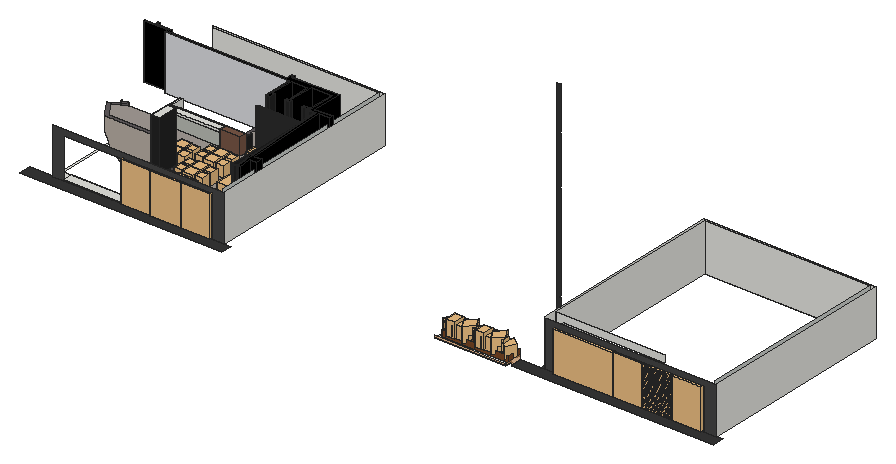
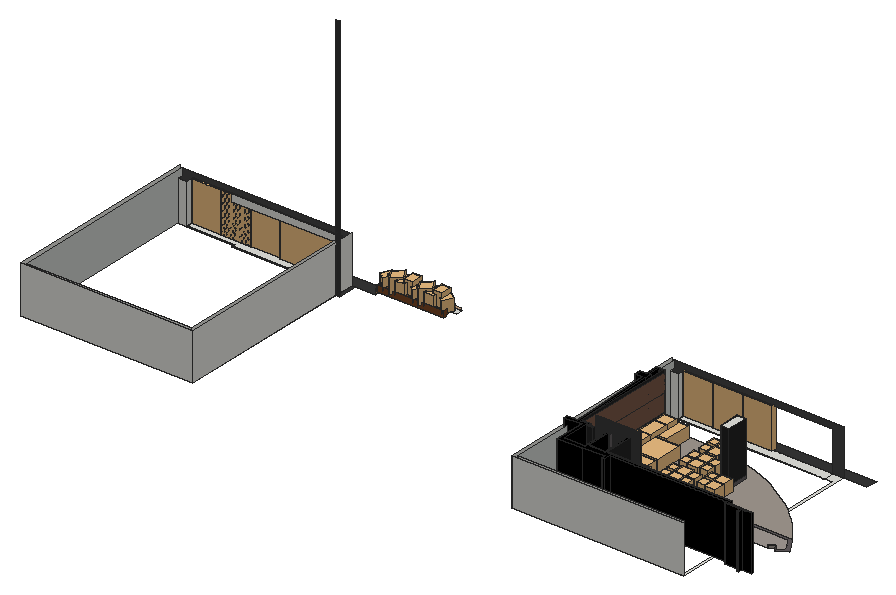
# SketchUp Ruby script. Lengths in inches.
U = 1.inch
M = Sketchup.active_model
def pt(a) = Geom::Point3d.new(a.map { |v| v * U })
def face(e, loops, mat)
  f = e.add_face(loops[0].map { |a| pt(a) })
  loops[1..].each { |l| e.add_face(l.map { |a| pt(a) }).erase! }
  f.material = f.back_material = mat if mat
  f
end
# faces: each face lists its corners as indices into pts; further lists are holes
def faces(e, pts, list, mat = nil) = list.each { |f| face(e, (f[0].is_a?(Array) ? f : [f]).map { |l| l.map { |i| pts[i] } }, mat) }
# xy, xz, yz: faces in a plane at the given z, y or x. An outline is a flat list of corners, or four numbers for a rectangle; further outlines are holes
def ring(l) = l.size == 4 ? [[l[0], l[1]], [l[2], l[1]], [l[2], l[3]], [l[0], l[3]]] : l.each_slice(2).to_a
def flat(e, list, mat, &to3) = list.each { |f| face(e, (f[0].is_a?(Array) ? f : [f]).map { |l| ring(l).map { |u, v| to3.(u, v) } }, mat) }
def xy(e, z, list, mat = nil) = flat(e, list, mat) { |x, y| [x, y, z] }
def xz(e, y, list, mat = nil) = flat(e, list, mat) { |x, z| [x, y, z] }
def yz(e, x, list, mat = nil) = flat(e, list, mat) { |y, z| [x, y, z] }
def lines(e, pts, list) = list.each { |a, b| e.add_line(pt(pts[a]), pt(pts[b])) }
# prism: a flat outline (further loops are holes) pulled along v
def prism(e, loops, v, mat = nil)
  f = face(e, loops, mat); d = Geom::Vector3d.new(v.map { |x| x * U })
  f.pushpull(f.normal.samedirection?(d) ? d.length : -d.length)
end
def box(e, o, s, mat = nil) = prism(e, [[o, [o[0] + s[0], o[1], o[2]], [o[0] + s[0], o[1] + s[1], o[2]], [o[0], o[1] + s[1], o[2]]]], [0, 0, s[2]], mat)
def at(x, y, z, deg = 0) = Geom::Transformation.translation(pt([x, y, z])) * Geom::Transformation.rotation(ORIGIN, Z_AXIS, deg.degrees)
def axes(o, x, y, z) = Geom::Transformation.new([*x, 0, *y, 0, *z, 0, *pt(o).to_a, 1])
def part(name) = M.definitions.add(name)
# library, detail: a bought-in or finely detailed component or shape, given as its bounding box
def library(name, o, s) = part(name).tap { |d| box(d.entities, o, s) }
def detail(e, o, s) = box(e.add_group.entities, o, s)
def put(e, d, t, mat = nil) = e.add_instance(d, t).tap { |i| i.material = mat if mat }
def group(e, t, mat = nil) = e.add_group.tap { |g| g.transformation = t; g.material = mat if mat }.entities
root = M.entities
M.materials.add("Biselado").color = [218, 219, 223]
M.materials.add("Concrete").color = [186, 188, 181]
M.materials.add("Floor board").color = [119, 86, 70]
M.materials.add("Floor board2").color = [119, 86, 70]
M.materials.add("Material__1").color = [95, 70, 46]
M.materials.add("Plastic Black ").color = [43, 43, 43]
M.materials.add("Screen Shot 2014-10-30 at 12.13.07").color = [162, 155, 149]
M.materials.add("Sophie_Shoes2").color = [35, 35, 35]
M.materials.add("Sophie_Skirt").color = [0, 0, 0]
M.materials.add("Untitsled-1").color = [96, 91, 93]
M.materials.add("Wood_Grain_Dark").color = [51, 47, 43]
M.materials.add("[Basic Tile]").color = [203, 206, 202]
M.materials.add("[Color_000]").color = [255, 255, 255]
M.materials.add("[Granite Dark Gray]").color = [69, 68, 68]
M.materials.add("[Metal_Corrogated_Shiny]2").color = [193, 193, 193]
M.materials.add("[Slate Light Tile]").color = [54, 54, 54]
M.materials.add("[Wood Floor]").color = [224, 152, 88]
M.materials["[Wood Floor]"].alpha = 0.68
M.materials.add("[Wood Veneer 01]").color = [120, 70, 37]
M.materials.add("t_planksnew0027_5_l_seamless_298 copy").color = [161, 153, 144]
c1 = library("Square table",[5.01,5.91,-0.2],[27.56,27.56,29.53])
c2 = library("ch24 wishbone chair by Carl Hansen & Son",[0,0,0],[21.1,19.68,29.02])
c3 = library("Scandinavian Door w/ Glass Wall\#2",[-41.94,78.85,0],[6.47,62.99,82.68])
c4 = part("Group\#72")
box(c4.entities,[0,-0.59,0],[31.5,1.77,87.4],"Sophie_Shoes2")
c5 = library("Armless sofa",[0,0,0],[31.59,51.18,39.76])
c6 = library("Sofa corner unit",[0,0,0],[31.57,31.52,39.76])
c7 = part("Group\#13")
box(c7.entities,[-0.79,0,0],[1.97,3.15,131.5],"Wood_Grain_Dark")
c8 = library("Group\#91",[-37.8,-0.03,0],[93.74,69.5,29.53])
c9 = library("Group\#68",[-37.8,-0.03,0],[93.74,69.5,29.53])
c10 = library("Group\#95",[0,-0.03,0],[55.94,69.5,29.53])
c11 = library("Areca palm plant",[0,0,0],[49.1,36.6,54.46])
c12 = library("Group\#440",[-84.69,-90.07,-0.36],[176.51,175.13,171.4])
c13 = library("Group\#441",[-7.34,-1.2,0],[38.67,35.81,49.04])
c14 = library("Group38\#2",[14.01,28.44,-23.43],[18.58,18.32,38.89])
c15 = library("Group20\#1",[-20.81,-17.08,3.79],[39.86,39.43,37.51])
c16 = part("Group\#443")
put(c16.entities,c11,axes([76.39,-6.2,6.08],[0.56191,0.45017,0],[-0.52986,0.66137,0],[0,0,0.72]))
put(c16.entities,c11,axes([178.2,-6.2,6.08],[0.56191,0.45017,0],[-0.52986,0.66137,0],[0,0,0.72]))
put(c16.entities,c12,axes([163.5,14.93,6.05],[0.08593,-0.04961,0],[0.04961,0.08593,0],[0,0,0.10522]))
put(c16.entities,c13,axes([144.89,24.9375,8],[-0.79,0,0],[0,-0.79,0],[0,0,0.79]))
put(c16.entities,c12,axes([113.57,17.19,6.07],[0.14087,-0.08133,0],[0.08133,0.14087,0],[0,0,0.1725]))
put(c16.entities,c14,axes([235.95,-4.1,28.17],[0,0.8848,0],[-0.94674,0,0],[0,0,0.85826]))
put(c16.entities,c12,axes([190.75,14.93,6.05],[0.08593,-0.04961,0],[0.04961,0.08593,0],[0,0,0.10522]))
put(c16.entities,c12,axes([61.68,14.93,6.05],[0.08593,-0.04961,0],[0.04961,0.08593,0],[0,0,0.10522]))
put(c16.entities,c12,axes([88.93,14.93,6.05],[0.08593,-0.04961,0],[0.04961,0.08593,0],[0,0,0.10522]))
put(c16.entities,c15,axes([154.82,18.97,4.77],[-0.85,0,0],[0,-0.85,0],[0,0,0.85]))
put(c16.entities,c12,axes([41.62,14.93,6.05],[0.08593,-0.04961,0],[0.04961,0.08593,0],[0,0,0.10522]))
put(c16.entities,c12,axes([143.43,14.93,6.05],[0.08593,-0.04961,0],[0.04961,0.08593,0],[0,0,0.10522]))
put(c16.entities,c14,axes([134.14,-4.1,28.17],[0,0.8848,0],[-0.94674,0,0],[0,0,0.85826]))
g1 = group(c16.entities,at(234.8,0,0,90),"[Wood Veneer 01]")
xy(g1,0,[[0,0,6,234.8],[30,0,36,234.8]])
xy(g1,3,[[6,0,30,234.8]])
xy(g1,7,[[6,5,30,229.8]],"Material__1")
xy(g1,15,[[[0,0,36,234.8],[6,5,30,229.8]]])
xz(g1,0,[[0,0,6,0,6,3,30,3,30,0,36,0,36,15,0,15]])
xz(g1,5,[[6,7,30,15]])
xz(g1,229.8,[[6,7,30,15]])
xz(g1,234.8,[[0,0,0,15,36,15,36,0,30,0,30,3,6,3,6,0]])
yz(g1,0,[[0,0,234.8,15]])
yz(g1,6,[[0,0,234.8,3],[5,7,229.8,15]])
yz(g1,30,[[0,0,234.8,3],[5,7,229.8,15]])
yz(g1,36,[[0,0,234.8,15]])
put(c16.entities,c13,axes([43.08,24.9375,8],[-0.79,0,0],[0,-0.79,0],[0,0,0.79]))
put(c16.entities,c12,axes([11.76,17.19,6.07],[0.14087,-0.08133,0],[0.08133,0.14087,0],[0,0,0.1725]))
put(c16.entities,c15,axes([53.01,18.97,4.77],[-0.85,0,0],[0,-0.85,0],[0,0,0.85]))
put(c16.entities,c12,axes([219.01,17.19,6.07],[0.14087,-0.08133,0],[0.08133,0.14087,0],[0,0,0.1725]))
xy(root,148.4375,[[3053.01,589.17,3053.01,1096.5,3491.44,1096.5,3491.44,589.17,3457.61,589.17,3457.61,608.75,3480.67,608.75,3480.67,1090.24,3059.27,1090.24,3059.27,616,3079.62,616,3079.62,589.17],[3079.62,589.17,3079.62,616,3336.64,616,3336.64,608.75,3457.61,608.75,3457.61,589.17],[4303.63,589.17,4303.63,1096.5,4742.06,1096.5,4742.06,589.17,4708.23,589.17,4708.23,608.75,4731.3,608.75,4731.3,1090.24,4309.9,1090.24,4309.9,616,4330.25,616,4330.25,589.17],[4330.25,589.17,4330.25,616,4587.26,616,4587.26,608.75,4708.23,608.75,4708.23,589.17]])
xy(root,148.4375,[[2993.46,559.875,3506.75,589.17],[4244.09,559.875,4757.37,589.17],[4294.9,589.17,4303.63,640.11]],"[Slate Light Tile]")
xy(root,149.625,[[3079.62,589.17,3457.61,589.17,3457.61,608.75,3336.64,608.75,3336.64,616,3079.62,616],[4330.25,589.17,4708.23,589.17,4708.23,608.75,4587.26,608.75,4587.26,616,4330.25,616]])
xy(root,155.3125,[[4061.87,542.125,4244.09,559.875]])
xz(root,542.125,[[4061.87,155.3125,4244.09,161.375]],"[Wood Floor]")
xz(root,589.17,[[3079.62,148.4375,3336.64,149.625],[3336.64,148.4375,3457.61,149.625],[4330.25,148.4375,4587.26,149.625],[4587.26,148.4375,4708.23,149.625]])
xz(root,589.17,[[3053.01,148.4375,3079.62,148.4375,3079.62,251.46,3457.61,251.46,3457.61,148.4375,3491.44,148.4375,3491.44,265.8125,3053.01,265.8125],[4303.63,148.4375,4330.25,148.4375,4330.25,251.46,4708.23,251.46,4708.23,148.4375,4742.06,148.4375,4742.06,265.8125,4303.63,265.8125]],"[Granite Dark Gray]")
xz(root,608.75,[[3336.64,148.4375,3457.61,149.625],[3457.61,148.4375,3480.67,251.46],[4587.26,148.4375,4708.23,149.625],[4708.23,148.4375,4731.3,251.46]])
xz(root,616,[[3079.62,148.4375,3336.64,149.625],[4309.9,148.4375,4309.9,268.4375,4587.26,268.4375,4587.26,251.46,4330.25,251.46,4330.25,148.4375],[4330.25,148.4375,4587.26,149.625]])
xz(root,640.11,[[4294.9,148.4375,4303.63,148.4375,4303.63,289.5625,4300.2,289.5625,4300.2,293,4303.63,293,4303.63,410.625,4301.7,410.625,4301.7,413.5,4303.63,413.5,4303.63,538.1875,4301.88,538.1875,4301.88,541.1875,4303.63,541.1875,4303.63,662.4375,4301.76,662.4375,4301.76,665.9375,4303.63,665.9375,4303.63,776.0625,4294.9,776.0625]],"[Slate Light Tile]")
xz(root,1090.24,[[3059.27,148.4375,3480.67,268.4375],[4309.9,148.4375,4731.3,268.4375]])
xz(root,1096.5,[[3053.01,148.4375,3491.44,268.4375],[4303.63,148.4375,4742.06,268.4375]])
yz(root,3336.64,[[608.75,148.4375,616,149.625]])
yz(root,3457.61,[[589.17,148.4375,608.75,149.625],[589.17,149.625,608.75,251.46]])
yz(root,3480.67,[[608.75,148.4375,608.75,251.46,595.44,251.46,595.44,268.4375,1090.24,268.4375,1090.24,148.4375]],"[Basic Tile]")
yz(root,3491.44,[[589.17,148.4375,1096.5,268.4375]])
yz(root,4244.09,[[559.875,148.4375,589.17,148.4375,589.17,161.375,542.125,161.375,542.125,155.3125,559.875,155.3125]],"[Wood Floor]")
yz(root,4303.63,[[589.17,148.4375,640.11,268.4375],[640.11,148.4375,1096.5,268.4375]])
yz(root,4309.9,[[616,148.4375,1090.24,268.4375]])
yz(root,4330.25,[[589.17,148.4375,616,149.625],[589.17,149.625,616,251.46]])
yz(root,4587.26,[[608.75,148.4375,616,149.625]])
yz(root,4708.23,[[589.17,148.4375,608.75,149.625],[589.17,149.625,608.75,251.46]])
yz(root,4731.3,[[608.75,148.4375,608.75,251.46,595.44,251.46,595.44,268.4375,1090.24,268.4375,1090.24,148.4375]],"[Basic Tile]")
yz(root,4742.06,[[589.17,148.4375,1096.5,268.4375]])
p = [[3382.97,998.54,148.89],[3382.97,998.73,148.89],[3464.42,662.13,148.89],[3464.46,662.13,148.89],[3451.42,661.28,148.89],[3451.42,661.28,235.5]]
lines(root,p,[[0,1],[2,3],[4,5]])
g2 = group(root,at(3111.07,900.11,148.89))
g3 = group(g2,at(0,0,0))
box(g3,[-5.91,0,0],[163.69,19.69,31.5])
g4 = group(root,at(2948.875,845,148.89),"Untitsled-1")
xy(g4,0,[[30.66,0,22.97,10.41,13.17,25.17,0,47.23,25.07,61.99,28.66,54.97,10.82,44.46,19.84,29.37,29.42,14.93,34.63,7.875,502.55,7.875,502.55,0],[29.6875,52.96,28.66,54.97,25.07,61.99,25.45,62.21,29.03,55.19,29.87,53.55,30.06,53.17],[150.39,55.12,162.2,61.02]])
xy(g4,0,[[34.63,7.875,29.42,14.93,19.84,29.37,10.82,44.46,28.66,54.97,29.6875,52.96,30.06,53.17,43.36,60.59,43.25,60.59,43.25,61.02,150.39,61.02,150.39,55.12,295.57,55.12,295.57,74.8,303.44,74.8,303.44,147.64,382.18,147.64,382.18,74.8,392.39,74.8,392.39,88.58,388.09,88.58,388.09,147.64,428.18,147.64,428.18,88.58,423.88,88.58,423.88,82.68,436.24,82.68,436.24,88.58,434.09,88.58,434.09,153.54,485.64,153.54,485.64,88.58,467.74,88.58,467.74,82.68,480.91,82.68,480.91,79.03,503.34,79.03,503.34,31.5,502.55,31.5,502.55,7.875]],"Screen Shot 2014-10-30 at 12.13.07")
xy(g4,0,[[295.57,74.8,303.44,147.64]],"Untitsled-1")
xy(g4,7.875,[[29.6875,52.96,25.07,61.99,25.45,62.21,29.03,55.19,29.87,53.55,43.25,61.02,43.25,60.59,43.36,60.59]],"Untitsled-1")
xz(g4,60.59,[[43.25,0,43.36,7.875]],"Screen Shot 2014-10-30 at 12.13.07")
yz(g4,43.25,[[60.59,0,61.02,7.875]],"Screen Shot 2014-10-30 at 12.13.07")
p = [[29.6875,52.96,7.875],[25.07,61.99,7.875],[25.07,61.99,0],[28.66,54.97,0],[29.6875,52.96,0],[30.06,53.17,0],
  [43.36,60.59,0],[43.36,60.59,7.875],[29.87,53.55,0],[29.03,55.19,0],[29.03,55.19,7.875],[29.87,53.55,7.875],
  [43.25,61.02,0],[43.25,61.02,7.875],[25.45,62.21,0],[25.45,62.21,7.875],[150.39,55.12,0],[150.39,39.37,0],
  [502.55,0,0],[503.34,0,0],[29.44,55.42,0],[43.45,60.64,0],[25.07,62,0],[502.55,78.21,0],
  [480.91,78.21,0],[480.91,79.03,0],[303.44,147.64,0],[303.44,155.51,0]]
faces(g4,p,[[0,1,2,3,4],[4,5,6,7,0],[8,9,10,11],[9,14,15,10],[14,2,1,15]])
faces(g4,p,[[8,12,13,11]],"Screen Shot 2014-10-30 at 12.13.07")
lines(g4,p,[[16,17],[18,19],[20,9],[6,21],[22,2],[23,24],[24,25],[26,27]])
g5 = group(g4,at(388.09,147.64,0))
xy(g5,0,[[0,-59.06,4.3,-59.06,4.3,-58.62,0.43,-58.62,0.43,-0.43,39.67,-0.43,39.67,-58.62,35.8,-58.62,35.8,-59.06,40.1,-59.06,40.1,0,0,0]],"Screen Shot 2014-10-30 at 12.13.07")
xy(g5,7.875,[[0,-59.06,0,-0.43,0.43,-0.43,0.43,-58.62,4.3,-58.62,4.3,-59.06],[35.8,-59.06,35.8,-58.62,39.67,-58.62,39.67,-0.43,40.1,-0.43,40.1,-59.06]],"Untitsled-1")
xy(g5,47.24,[[0,-0.43,40.1,0]],"Untitsled-1")
xz(g5,-59.06,[[35.8,0,40.1,7.875]],"Screen Shot 2014-10-30 at 12.13.07")
xz(g5,-59.06,[[0,0,4.3,7.875]],"Untitsled-1")
xz(g5,-58.62,[[0.43,0,4.3,7.875],[35.8,0,39.67,7.875]],"Untitsled-1")
xz(g5,-0.43,[[0,7.875,40.1,39.37]],"Screen Shot 2014-10-30 at 12.13.07")
xz(g5,-0.43,[[0.43,0,39.67,7.875],[0,39.37,40.1,47.24]],"Untitsled-1")
yz(g5,0,[[-59.06,0,0,0,0,39.37,-0.43,39.37,-0.43,7.875,-59.06,7.875]],"Screen Shot 2014-10-30 at 12.13.07")
yz(g5,0,[[-0.43,39.37,0,47.24]],"Untitsled-1")
yz(g5,0.43,[[-58.62,0,-0.43,7.875]],"Untitsled-1")
yz(g5,4.3,[[-59.06,0,-58.62,7.875]],"Untitsled-1")
yz(g5,35.8,[[-59.06,0,-58.62,7.875]],"Untitsled-1")
yz(g5,39.67,[[-58.62,0,-0.43,7.875]],"Untitsled-1")
yz(g5,40.1,[[-59.06,0,-59.06,7.875,-0.43,7.875,-0.43,39.37,0,39.37,0,0]],"Screen Shot 2014-10-30 at 12.13.07")
yz(g5,40.1,[[-0.43,39.37,0,47.24]],"Untitsled-1")
g6 = group(g4,at(434.09,153.54,0))
xy(g6,0,[[0,-64.96,2.15,-64.96,2.15,-64.53,0.43,-64.53,0.43,-0.43,51.11,-0.43,51.11,-64.53,33.65,-64.53,33.65,-64.96,51.55,-64.96,51.55,0,0,0]],"Screen Shot 2014-10-30 at 12.13.07")
xy(g6,7.875,[[0,-64.96,0,-0.43,0.43,-0.43,0.43,-64.53,2.15,-64.53,2.15,-64.96],[33.65,-64.96,33.65,-64.53,51.11,-64.53,51.11,-0.43,51.55,-0.43,51.55,-64.96]],"Untitsled-1")
xy(g6,47.24,[[0,-0.43,51.55,0]],"Untitsled-1")
xz(g6,-64.96,[[0,0,2.15,7.875],[33.65,0,51.55,7.875]],"Untitsled-1")
xz(g6,-64.53,[[0.43,0,2.15,7.875],[33.65,0,51.11,7.875]],"Untitsled-1")
xz(g6,-0.43,[[0,7.875,51.55,39.37]],"Screen Shot 2014-10-30 at 12.13.07")
xz(g6,-0.43,[[0.43,0,51.11,7.875],[0,39.37,51.55,47.24]],"Untitsled-1")
xz(g6,0,[[40.1,0,51.55,39.37]],"Screen Shot 2014-10-30 at 12.13.07")
xz(g6,0,[[40.1,39.37,51.55,47.24]],"Untitsled-1")
yz(g6,0,[[-64.96,0,0,0,0,39.37,-0.43,39.37,-0.43,7.875,-64.96,7.875]],"Screen Shot 2014-10-30 at 12.13.07")
yz(g6,0,[[-0.43,39.37,0,47.24]],"Untitsled-1")
yz(g6,0.43,[[-64.53,0,-0.43,7.875]],"Untitsled-1")
yz(g6,2.15,[[-64.96,0,-64.53,7.875]],"Untitsled-1")
yz(g6,33.65,[[-64.96,0,-64.53,7.875]],"Untitsled-1")
yz(g6,51.11,[[-64.53,0,-0.43,7.875]],"Untitsled-1")
yz(g6,51.55,[[-64.96,0,-64.96,7.875,-0.43,7.875,-0.43,39.37,0,39.37,0,0]],"Screen Shot 2014-10-30 at 12.13.07")
yz(g6,51.55,[[-0.43,39.37,0,47.24]],"Untitsled-1")
put(root,c1,at(3223.26,766.11,148.89,89.836))
put(root,c1,at(3223.26,794.18,148.89,89.836))
g7 = group(root,at(3202.39,714.02,148.89))
xy(g7,0,[[-0.59,-0.59,22.24,53.74]])
xy(g7,7.875,[[-0.59,-0.59,22.24,0],[-0.59,0,0,53.15],[21.65,0,22.24,53.15],[-0.59,53.15,22.24,53.74]],"Untitsled-1")
xy(g7,137.44,[[0,0,21.65,53.15]])
xz(g7,-0.59,[[-0.59,0,22.24,7.875]],"Untitsled-1")
xz(g7,0,[[0,7.875,21.65,137.44]],"Sophie_Shoes2")
xz(g7,53.15,[[0,7.875,21.65,137.44]],"Sophie_Shoes2")
xz(g7,53.74,[[-0.59,0,22.24,7.875]],"Untitsled-1")
yz(g7,-0.59,[[-0.59,0,53.74,7.875]],"Untitsled-1")
yz(g7,0,[[0,7.875,53.15,137.44]],"Sophie_Shoes2")
yz(g7,21.65,[[0,7.875,53.15,137.44]],"Sophie_Shoes2")
yz(g7,22.24,[[-0.59,0,53.74,7.875]],"Untitsled-1")
g8 = group(root,at(2952.73,661.35,148.89))
xy(g8,0,[[511.73,0,511.7,0.79,510.27,31.46,508.31,31.46,507.48,49.07,509.45,49.07,499.49,263.4,481.79,262.65,481.79,265.89,463.89,265.89,463.89,272.23,481.79,272.23,481.79,337.19,430.24,337.19,430.24,272.23,432.39,272.23,432.39,265.89,420.03,265.89,420.03,272.23,424.33,272.23,424.33,331.29,384.24,331.29,384.24,272.23,388.54,272.23,388.54,258.02,377.9,258.02,377.9,331.29,62.06,331.29,62.06,341.13,1.14,341.13,0,345.07,25.02,345.07,25.02,355.33,28.95,355.33,28.95,347.03,67.96,347.03,67.96,339.16,365.84,339.16,365.84,355.33,373.72,355.33,373.72,346.57,430.24,349.18,491.63,352.02,491.63,272.99,534.09,274.79,534.09,264.94,507.35,263.81,517.3125,49.53,534.09,50.31,534.09,32.57,518.14,31.83,519.6,0.37,514.8125,0]],"Sophie_Skirt")
xy(g8,7.875,[[377.9,258.02,378.33,331.29],[378.33,258.02,388.54,258.45],[420.03,265.89,432.39,266.33],[463.89,265.89,481.79,266.33]],"Untitsled-1")
xy(g8,137.8,[[511.73,0,514.8125,0,519.6,0.37,518.14,31.83,534.09,32.57,534.09,50.31,517.3125,49.53,507.35,263.81,534.09,264.94,534.09,274.79,491.63,272.99,491.63,352.02,430.24,349.18,373.72,346.57,373.72,355.33,365.84,355.33,365.84,339.16,67.96,339.16,67.96,347.03,28.95,347.03,28.95,355.33,25.02,355.33,25.02,345.07,0,345.07,1.14,341.13,62.06,341.13,62.06,331.29,378.33,331.29,378.33,258.45,388.54,258.45,388.54,272.23,384.24,272.23,384.24,331.29,424.33,331.29,424.33,272.23,420.03,272.23,420.03,266.33,432.39,266.33,432.39,272.23,430.24,272.23,430.24,337.19,481.79,337.19,481.79,272.23,463.89,272.23,463.89,266.33,481.79,266.33,481.79,262.65,499.49,263.4,509.45,49.07,507.48,49.07,508.31,31.46,510.27,31.46,511.7,0.79]],"Sophie_Skirt")
xz(g8,0,[[511.73,0,514.8125,137.8]],"Sophie_Skirt")
xz(g8,31.46,[[508.31,0,510.27,137.8]],"Sophie_Skirt")
xz(g8,49.07,[[507.48,0,509.45,137.8]],"Sophie_Skirt")
xz(g8,258.02,[[377.9,0,388.54,7.875]],"Untitsled-1")
xz(g8,258.45,[[378.33,7.875,388.54,137.8]],"Sophie_Shoes2")
xz(g8,265.89,[[420.03,0,432.39,7.875],[463.89,0,481.79,7.875]],"Untitsled-1")
xz(g8,266.33,[[420.03,7.875,432.39,137.8],[463.89,7.875,481.79,137.8]],"Sophie_Shoes2")
xz(g8,272.23,[[384.24,0,388.54,137.8],[420.03,0,424.33,137.8],[430.24,0,432.39,137.8],[463.89,0,481.79,137.8]],"Sophie_Shoes2")
xz(g8,331.29,[[62.06,0,377.9,0,377.9,7.875,378.33,7.875,378.33,137.8,62.06,137.8]],"Biselado")
xz(g8,331.29,[[384.24,0,424.33,137.8]],"Sophie_Skirt")
xz(g8,337.19,[[430.24,0,481.79,137.8]],"Sophie_Skirt")
xz(g8,339.16,[[67.96,0,365.84,137.8]],"Sophie_Skirt")
xz(g8,341.13,[[1.14,0,62.06,137.8]],"Sophie_Skirt")
xz(g8,345.07,[[0,0,25.02,137.8]],"Sophie_Skirt")
xz(g8,347.03,[[28.95,0,67.96,137.8]],"Sophie_Skirt")
xz(g8,355.33,[[25.02,0,28.95,137.8],[365.84,0,373.72,137.8]],"Sophie_Skirt")
yz(g8,25.02,[[345.07,0,355.33,137.8]],"Sophie_Skirt")
yz(g8,28.95,[[347.03,0,355.33,137.8]],"Sophie_Skirt")
yz(g8,62.06,[[331.29,0,341.13,137.8]],"Sophie_Skirt")
yz(g8,67.96,[[339.16,0,347.03,137.8]],"Sophie_Skirt")
yz(g8,365.84,[[339.16,0,355.33,137.8]],"Sophie_Skirt")
yz(g8,373.72,[[346.57,0,355.33,137.8]],"Sophie_Skirt")
yz(g8,377.9,[[258.02,0,331.29,7.875]],"Untitsled-1")
yz(g8,378.33,[[258.45,7.875,331.29,137.8]],"Sophie_Shoes2")
yz(g8,384.24,[[272.23,0,331.29,137.8]],"Sophie_Skirt")
yz(g8,388.54,[[258.02,0,272.23,0,272.23,137.8,258.45,137.8,258.45,7.875,258.02,7.875]],"Sophie_Shoes2")
yz(g8,420.03,[[265.89,0,265.89,7.875,266.33,7.875,266.33,137.8,272.23,137.8,272.23,0]],"Untitsled-1")
yz(g8,424.33,[[272.23,0,331.29,137.8]],"Sophie_Skirt")
yz(g8,430.24,[[272.23,0,337.19,137.8]],"Sophie_Skirt")
yz(g8,432.39,[[265.89,0,272.23,0,272.23,137.8,266.33,137.8,266.33,7.875,265.89,7.875]],"Sophie_Shoes2")
yz(g8,463.89,[[265.89,0,265.89,7.875,266.33,7.875,266.33,137.8,272.23,137.8,272.23,0]],"Sophie_Shoes2")
yz(g8,481.79,[[262.65,0,262.65,137.8,266.33,137.8,266.33,7.875,265.89,7.875,265.89,0],[272.23,0,337.19,137.8]],"Sophie_Skirt")
yz(g8,491.63,[[272.99,0,352.02,137.8]],"Sophie_Skirt")
yz(g8,534.09,[[32.57,0,50.31,137.8],[264.94,0,274.79,137.8]],"Sophie_Skirt")
p = [[511.7,0.79,0],[511.73,0,0],[511.73,0,137.8],[511.7,0.79,137.8],[514.8125,0,0],[519.6,0.37,0],
  [519.6,0.37,137.8],[514.8125,0,137.8],[518.14,31.83,0],[518.14,31.83,137.8],[510.27,31.46,0],[510.27,31.46,137.8],
  [507.48,49.07,0],[508.31,31.46,0],[508.31,31.46,137.8],[507.48,49.07,137.8],[534.09,32.57,0],[534.09,32.57,137.8],
  [499.49,263.4,0],[509.45,49.07,0],[509.45,49.07,137.8],[499.49,263.4,137.8],[517.3125,49.53,0],[507.35,263.81,0],
  [507.35,263.81,137.8],[517.3125,49.53,137.8],[534.09,50.31,0],[534.09,50.31,137.8],[481.79,262.65,0],[481.79,262.65,137.8],
  [534.09,264.94,0],[534.09,264.94,137.8],[534.09,274.79,0],[491.63,272.99,0],[491.63,272.99,137.8],[534.09,274.79,137.8],
  [0,345.07,0],[1.14,341.13,0],[1.14,341.13,137.8],[0,345.07,137.8],[430.24,349.18,0],[373.72,346.57,0],
  [373.72,346.57,137.8],[430.24,349.18,137.8],[491.63,352.02,0],[491.63,352.02,137.8]]
faces(g8,p,[[0,1,2,3],[4,5,6,7],[5,8,9,6],[10,0,3,11],[12,13,14,15],[8,16,17,9],[18,19,20,21],[22,23,24,25],
  [26,22,25,27],[28,18,21,29],[23,30,31,24],[32,33,34,35],[36,37,38,39],[40,41,42,43],[44,40,43,45]],"Sophie_Skirt")
g9 = group(g8,at(146.54,223.02,0))
xy(g9,0,[[0,0,0,51.18,5.91,51.18,5.91,16.93,145.18,16.93,145.18,6.69,5.91,6.69,5.91,0]],"Concrete")
xy(g9,37.4,[[5.91,0,145.18,6.69]])
xy(g9,43.31,[[0,0,145.18,0,145.18,16.93,5.91,16.93,5.91,51.18,0,51.18]])
xz(g9,0,[[0,0,5.91,0,5.91,37.4,145.18,37.4,145.18,43.31,0,43.31]])
xz(g9,6.69,[[5.91,36.8125,6.5,36.8125,10.63,37.4,5.91,37.4]])
xz(g9,6.69,[[5.91,0,5.91,36.8125,6.5,36.8125,10.63,37.4,145.18,37.4,145.18,0]],"Concrete")
xz(g9,16.93,[[5.91,0,145.18,43.31]],"[Color_000]")
xz(g9,51.18,[[0,0,5.91,43.31]],"Concrete")
yz(g9,0,[[0,0,51.18,43.31]])
yz(g9,5.91,[[0,0,6.69,37.4],[16.93,0,51.18,43.31]])
yz(g9,145.18,[[6.69,0,16.93,0,16.93,43.31,0,43.31,0,37.4,6.69,37.4]],"Concrete")
p = [[190.45,16.14,0],[190.45,15.75,0],[169.59,16.14,0],[169.59,15.75,0]]
lines(g9,p,[[0,1],[2,3]])
g10 = group(root,at(2979.53,652.11,148.89),"t_planksnew0027_5_l_seamless_298 copy")
xy(g10,0,[[429.35,0,354.79,0.42,331.3,2.55,319.24,4.03,295.95,7.5625,272.9,12.11,229.52,24.41,206.75,33.49,183.99,42.57,173.49,47.99,162.94,53.43,103.01,90.75,94.03,97,85.51,104.03,76.98,111.05,63.55,122.79,50.29,134.84,37.79,147.5,24.1875,162.86,7,183.74,0,192.89,472.68,192.89,472.68,9.29,486.38,9.29,486.38,1.89]],"t_planksnew0027_5_l_seamless_298 copy")
put(root,c2,at(3220.15,823.08,148.89,-90.164))
put(root,c2,at(3220.15,796.07,148.89,-90.164))
put(root,c2,at(3269.64,727.93,148.89,89.836))
put(root,c2,at(3269.64,692.97,148.89,89.836))
put(root,c2,at(3269.64,754.94,148.89,89.836))
put(root,c2,at(3269.64,664.67,148.89,89.836))
put(root,c2,at(3269.64,794.74,148.89,89.836))
put(root,c2,at(3269.64,821.75,148.89,89.836))
g11 = group(root,at(3244.44,881.61,148.89))
g12 = group(g11,at(0,0,0))
xy(g12,1.97,[[24.41,37.01,25.2,37.4],[25.2,37.01,48.23,37.4]],"Sophie_Shoes2")
xy(g12,1.97,[[48.23,37.01,50,38.1875]],"Wood_Grain_Dark")
xy(g12,2.76,[[0,0,51.18,10.24],[25.2,19.69,48.23,37.4]],"Plastic Black ")
xy(g12,2.76,[[50,10.24,51.18,19.25]],"Wood_Grain_Dark")
xy(g12,13.58,[[25.2,19.69,48.23,37.01]],"Plastic Black ")
xy(g12,14.37,[[25.2,19.69,48.23,37.01]],"Plastic Black ")
xy(g12,25.98,[[25.2,19.69,48.23,37.4]],"Plastic Black ")
xy(g12,26.77,[[25.2,19.69,48.23,19.69,48.23,22.83,47.44,22.83,47.44,37.4,25.2,37.4]],"Plastic Black ")
xy(g12,27.6875,[[27.68,18.11,45.43,19.69]])
xy(g12,30.71,[[25.2,22.83,47.44,37.4]],"Plastic Black ")
xy(g12,31.23,[[27.68,18.11,45.43,19.69]])
xy(g12,31.5,[[24.41,19.69,25.2,19.69,25.2,22.83,48.23,22.83,48.23,37.4,24.41,37.4]],"Plastic Black ")
xy(g12,35.93,[[24.41,19.25,50,19.25,50,38.1875,48.23,38.1875,48.23,19.69,24.41,19.69]],"Sophie_Shoes2")
xy(g12,35.93,[[0,19.25,24.41,19.69]],"[Color_000]")
xy(g12,46.0625,[[0,0,51.18,19.25]],"Floor board2")
xz(g12,0,[[0,2.76,51.18,46.0625]],"Floor board2")
xz(g12,10.24,[[0,0,50,2.76]],"Plastic Black ")
xz(g12,18.11,[[27.68,27.6875,45.43,31.23]])
xz(g12,19.25,[[50,2.76,50,35.93,0,35.93,0,46.0625,51.18,46.0625,51.18,2.76]],"Floor board2")
xz(g12,19.69,[[25.2,2.76,48.23,13.58],[25.2,13.58,48.23,14.37],[25.2,14.37,48.23,25.98]],"Plastic Black ")
xz(g12,19.69,[[[25.2,26.77,25.2,31.5,24.41,31.5,24.41,35.93,48.23,35.93,48.23,26.77],[27.68,27.6875,45.43,31.23]]],"Sophie_Shoes2")
xz(g12,19.69,[[0,0,24.41,35.93]],"[Color_000]")
xz(g12,22.83,[[47.44,26.77,48.23,26.77,48.23,31.5,25.2,31.5,25.2,30.71,47.44,30.71]],"Plastic Black ")
xz(g12,37.01,[[25.2,13.58,48.23,14.37]],"Plastic Black ")
xz(g12,37.01,[[24.41,0,50,1.97]],"Sophie_Shoes2")
xz(g12,37.4,[[[24.41,1.97,24.41,31.5,48.23,31.5,48.23,25.98,25.2,25.98,25.2,2.76,48.23,2.76,48.23,1.97],[25.2,26.77,47.44,30.71]]],"Sophie_Shoes2")
xz(g12,38.1875,[[48.23,1.97,50,35.93]],"Plastic Black ")
yz(g12,0,[[10.24,0,10.24,2.76,0,2.76,0,46.0625,19.25,46.0625,19.25,0]],"Floor board2")
yz(g12,0,[[19.25,0,19.69,35.93]],"[Color_000]")
yz(g12,24.41,[[19.69,0,19.69,31.5,37.4,31.5,37.4,1.97,37.01,1.97,37.01,0]],"Plastic Black ")
yz(g12,25.2,[[19.69,2.76,37.4,13.58],[19.69,13.58,37.01,14.37],[19.69,14.37,37.4,25.98],[19.69,26.77,37.4,26.77,37.4,30.71,22.83,30.71,22.83,31.5,19.69,31.5]],"Plastic Black ")
yz(g12,25.2,[[37.01,13.58,37.4,14.37]],"Sophie_Shoes2")
yz(g12,27.68,[[18.11,27.6875,19.69,31.23]])
yz(g12,45.43,[[18.11,27.6875,19.69,31.23]])
yz(g12,47.44,[[22.83,26.77,37.4,30.71]],"Plastic Black ")
yz(g12,48.23,[[37.4,1.97,37.4,2.76,19.69,2.76,19.69,13.58,37.01,13.58,37.01,14.37,19.69,14.37,19.69,25.98,37.4,25.98,37.4,31.5,22.83,31.5,22.83,26.77,19.69,26.77,19.69,35.93,38.1875,35.93,38.1875,1.97],[19.69,13.58,37.01,14.37]],"Plastic Black ")
yz(g12,50,[[10.24,0,37.01,0,37.01,1.97,38.1875,1.97,38.1875,35.93,19.25,35.93,19.25,2.76,10.24,2.76]],"Sophie_Shoes2")
yz(g12,51.18,[[0,2.76,19.25,46.0625]],"Floor board2")
p = [[24.41,18.5,46.0625],[24.41,18.5,46.16],[0,8.86,37.4],[0,10.24,37.4]]
lines(g12,p,[[0,1],[2,3]])
put(root,c1,at(3266.54,721.86,148.89,-90.164))
put(root,c1,at(3266.54,784.9,148.89,-90.164))
put(root,c1,at(3266.54,693.79,148.89,-90.164))
put(root,c1,at(3266.54,756.82,148.89,-90.164))
put(root,c1,at(3266.54,851.71,148.89,-90.164))
put(root,c1,at(3266.54,823.64,148.89,-90.164))
put(root,c3,axes([3230.92,518.17,380.12],[0,-1.83,0],[0,0,-1.61667],[1.83,0,0]))
put(root,c2,axes([3303.22,754.94,148.89],[-0.00287,1,0],[1,0.00287,0],[0,0,1]))
put(root,c2,axes([3303.22,727.93,148.89],[-0.00287,1,0],[1,0.00287,0],[0,0,1]))
put(root,c2,axes([3303.22,664.67,148.89],[-0.00287,1,0],[1,0.00287,0],[0,0,1]))
put(root,c2,axes([3303.22,692.97,148.89],[-0.00287,1,0],[1,0.00287,0],[0,0,1]))
put(root,c2,axes([3303.22,821.75,148.89],[-0.00287,1,0],[1,0.00287,0],[0,0,1]))
put(root,c2,axes([3303.22,794.74,148.89],[-0.00287,1,0],[1,0.00287,0],[0,0,1]))
put(root,c4,at(3341.26,927.67,148.89))
put(root,c3,axes([3305.18,518.17,380.12],[0,-1.83,0],[0,0,-1.61667],[1.83,0,0]))
g13 = group(root,at(3362.63,652.5625,148.6875))
put(g13,c5,at(86.72,196.88,0,-180))
put(g13,c5,at(86.72,145.7,0,-180))
put(g13,c5,at(4.02,228.45,0,-90))
put(g13,c6,at(55.2,228.45,0,-90))
put(g13,c6,at(86.72,43.34,0,-180))
put(g13,c6,at(-27.56,196.93,0))
put(g13,c5,at(86.72,94.52,0,-180))
g14 = group(root,at(3340.04,881.22,148.89))
put(g14,c7,at(100,0,0))
put(g14,c7,at(57.48,0,0))
put(g14,c7,at(92.91,0,0))
put(g14,c7,at(7.875,0,0))
put(g14,c7,at(107.09,0,0))
put(g14,c7,at(103.54,0,0))
put(g14,c7,at(61.02,0,0))
put(g14,c7,at(29.13,0,0))
put(g14,c7,at(68.11,0,0))
put(g14,c7,at(22.05,0,0))
put(g14,c7,at(78.74,0,0))
put(g14,c7,at(14.96,0,0))
put(g14,c7,at(82.28,0,0))
put(g14,c7,at(71.65,0,0))
put(g14,c7,at(75.2,0,0))
put(g14,c7,at(25.59,0,0))
put(g14,c7,at(18.5,0,0))
put(g14,c7,at(43.31,0,0))
put(g14,c7,at(64.57,0,0))
put(g14,c7,at(53.9375,0,0))
put(g14,c7,at(85.83,0,0))
put(g14,c7,at(89.37,0,0))
put(g14,c7,at(11.42,0,0))
put(g14,c7,at(0.79,0,0))
put(g14,c7,at(4.33,0,0))
put(g14,c7,at(36.22,0,0))
put(g14,c7,at(39.76,0,0))
put(g14,c7,at(32.68,0,0))
put(g14,c7,at(96.46,0,0))
put(g14,c7,at(46.85,0,0))
put(g14,c7,at(50.39,0,0))
put(g14,c7,at(-2.76,0,0))
put(root,c4,at(3385.12,927.67,148.89))
put(root,c8,at(3393.02,733.4375,148.6875))
put(root,c9,at(3393.02,808.28,148.6875))
put(root,c10,at(3393.02,657.53,148.6875))
g15 = group(root,at(3434.51,661.35,148.89),"Sophie_Shoes2")
xy(g15,0,[[16.91,-1.18,16.91,-0.07,14.95,-0.07,14.95,222.49,16.91,222.49,16.91,261.27,-5.31,261.27,-5.31,266.33,-3.9375,266.33,-3.9375,262.65,17.7,262.65,17.7,223.02,18.5,223.02,18.5,0.79,29.91,0.79,29.95,0,29.95,-1.18]])
xy(g15,7.875,[[-5.31,261.27,-4.72,266.33],[-4.72,261.27,16.91,261.86]],"Untitsled-1")
xy(g15,36.61,[[15.34,0.32,16.91,222.1]])
xy(g15,39.37,[[14.95,-0.07,16.91,-0.07,16.91,0,17.7,0,17.7,261.86,16.91,261.86,16.91,0.32,15.34,0.32,15.34,222.1,16.91,222.1,16.91,222.49,14.95,222.49]])
xy(g15,40.55,[[16.91,0,17.7,223.02],[16.91,223.02,17.7,261.86]])
xy(g15,85.43,[[16.91,0,17.7,261.86]],"Floor board2")
xy(g15,86.61,[[16.91,0,17.7,261.86]])
xy(g15,131.5,[[16.91,-0.07,17.7,261.86]],"Floor board2")
xy(g15,137.8,[[17.7,-1.18,29.95,-1.18,29.95,0,29.91,0.79,18.5,0.79,18.5,223.02,17.7,223.02],[-4.72,261.86,17.7,261.86,17.7,262.65,-3.9375,262.65,-3.9375,266.33,-4.72,266.33]])
xy(g15,137.8,[[16.91,-1.18,17.7,-0.07]],"Sophie_Shoes2")
xz(g15,-1.18,[[16.91,0,29.95,137.8]],"Sophie_Shoes2")
xz(g15,-0.07,[[14.95,3.9375,16.91,39.37],[16.91,131.5,17.7,137.8]],"Sophie_Shoes2")
xz(g15,-0.07,[[14.95,0,16.91,3.9375]],"[Metal_Corrogated_Shiny]2")
xz(g15,0,[[16.91,39.37,17.7,40.55],[16.91,40.55,17.7,40.94],[16.91,85.43,17.7,86.61]])
xz(g15,0.32,[[15.34,36.61,16.52,39.37],[16.52,36.61,16.91,39.37]])
xz(g15,0.79,[[18.5,0,29.91,137.8]])
xz(g15,222.1,[[15.34,36.61,16.91,39.37]])
xz(g15,222.49,[[14.95,0,16.91,7.875],[14.95,7.875,16.91,39.37]],"Sophie_Shoes2")
xz(g15,261.27,[[-5.31,0,16.91,7.875]],"Untitsled-1")
xz(g15,261.86,[[16.91,39.37,17.7,39.76]])
xz(g15,261.86,[[-4.72,7.875,16.91,7.875,16.91,39.76,17.7,39.76,17.7,40.55,16.91,40.55,16.91,85.43,17.7,85.43,17.7,86.61,16.91,86.61,16.91,131.5,17.7,131.5,17.7,137.8,-4.72,137.8]],"Sophie_Shoes2")
xz(g15,262.65,[[-3.9375,0,17.7,137.8]])
xz(g15,266.33,[[-5.31,0,-5.31,7.875,-4.72,7.875,-4.72,137.8,-3.9375,137.8,-3.9375,0]])
yz(g15,-5.31,[[261.27,0,266.33,7.875]],"Untitsled-1")
yz(g15,-4.72,[[261.86,7.875,266.33,137.8]],"Sophie_Shoes2")
yz(g15,-3.9375,[[262.65,0,266.33,137.8]])
yz(g15,14.95,[[-0.07,3.9375,222.49,39.37]],"Sophie_Shoes2")
yz(g15,14.95,[[-0.07,0,222.49,3.9375]],"[Metal_Corrogated_Shiny]2")
yz(g15,15.34,[[0.32,36.61,222.1,39.37]])
yz(g15,16.91,[[0.32,36.61,222.1,39.37]])
yz(g15,16.91,[[0,40.55,0,40.94,-0.07,40.94,-0.07,86.61,0,86.61,0,85.43,261.86,85.43,261.86,40.55]],"Floor board")
yz(g15,16.91,[[-0.07,39.37,0,40.94],[-0.07,86.61,-0.07,131.5,261.86,131.5,261.86,87.4,232.86,87.4,232.86,86.61]],"Floor board2")
yz(g15,16.91,[[222.49,0,222.49,39.37,261.86,39.37,261.86,7.875,261.27,7.875,261.27,0]],"Screen Shot 2014-10-30 at 12.13.07")
yz(g15,16.91,[[-1.18,0,-0.07,40.94],[-1.18,40.94,-0.07,86.61],[-1.18,86.61,-0.07,137.8],[232.86,86.61,261.86,87.4]],"Sophie_Shoes2")
yz(g15,17.7,[[223.02,0,262.65,0,262.65,137.8,261.86,137.8,261.86,85.43,223.02,85.43,223.02,40.55,261.86,40.55,261.86,39.37,223.02,39.37],[0,39.37,261.86,40.55],[0,40.55,223.02,40.94],[0,85.43,261.86,86.61]])
yz(g15,17.7,[[-0.07,131.5,261.86,137.8]],"Sophie_Shoes2")
yz(g15,18.5,[[0.79,0,223.02,137.8]])
yz(g15,29.95,[[-1.18,0,0,137.8]])
p = [[29.95,0,0],[29.91,0.79,0],[29.91,0.79,137.8],[29.95,0,137.8],[16.91,261.86,105.12],[16.91,272.94,105.12],
  [16.91,49.92,72.44],[17.7,49.92,72.44],[16.91,0,72.44],[17.7,0,72.44],[17.7,0,105.12],[17.7,0.79,105.12],
  [16.91,49.92,105.12],[17.7,49.92,105.12],[16.91,0,105.12],[17.7,0.79,72.44],[16.52,0.32,39.37],[16.52,0.39,39.37],
  [17.31,0.39,39.37],[17.31,222.1,39.37],[17.31,261.47,39.37],[17.31,223.02,39.37],[16.91,222.1,39.37]]
faces(g15,p,[[0,1,2,3]])
lines(g15,p,[[4,5],[6,7],[8,9],[10,11],[12,13],[14,10],[15,7],[9,15],[16,17],[18,19],[20,21],[19,22],
  [21,19]])
put(root,c16,axes([4070.99,553.5,156.81],[0.72468,0,0],[0,1,0],[0,0,1]))
put(root,c3,axes([4330.25,518.89,378.93],[0,-1.83,0],[0,0,-1.61667],[1.83,0,0]))
put(root,c3,axes([4481.55,518.17,380.12],[0,-1.83,0],[0,0,-1.61667],[1.83,0,0]))
put(root,c3,axes([4555.81,518.17,380.12],[0,-1.83,0],[0,0,-1.61667],[1.83,0,0]))
